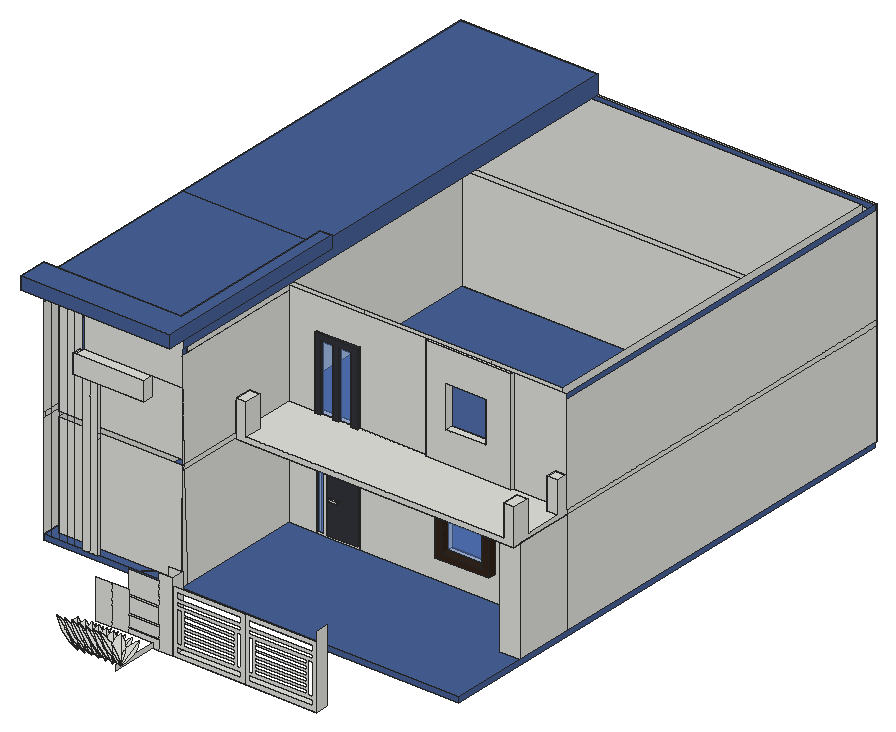
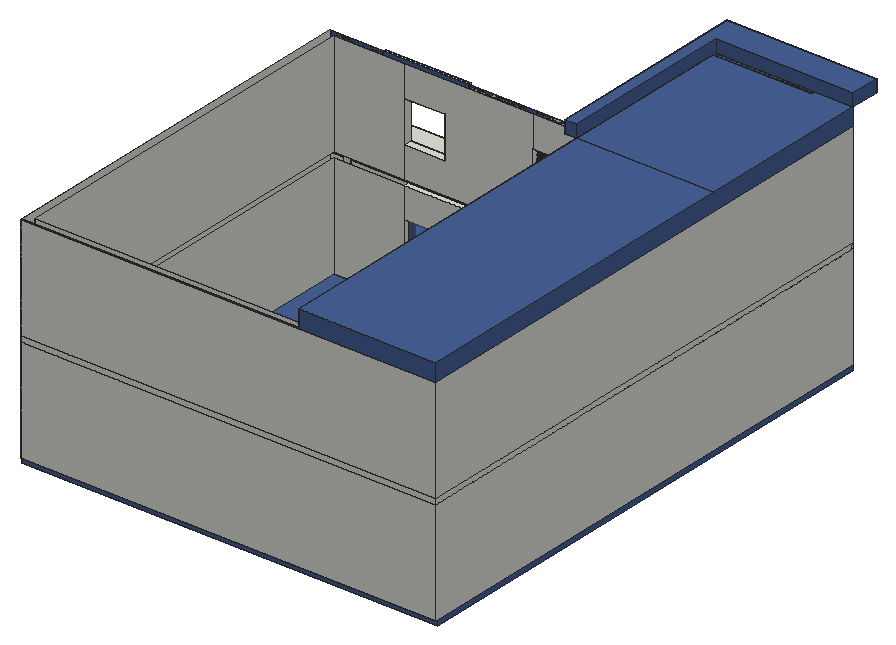
# SketchUp Ruby script. Lengths in inches.
U = 1.inch
M = Sketchup.active_model
def pt(a) = Geom::Point3d.new(a.map { |v| v * U })
def face(e, loops, mat)
  f = e.add_face(loops[0].map { |a| pt(a) })
  loops[1..].each { |l| e.add_face(l.map { |a| pt(a) }).erase! }
  f.material = f.back_material = mat if mat
  f
end
# faces: each face lists its corners as indices into pts; further lists are holes
def faces(e, pts, list, mat = nil) = list.each { |f| face(e, (f[0].is_a?(Array) ? f : [f]).map { |l| l.map { |i| pts[i] } }, mat) }
# xy, xz, yz: faces in a plane at the given z, y or x. An outline is a flat list of corners, or four numbers for a rectangle; further outlines are holes
def ring(l) = l.size == 4 ? [[l[0], l[1]], [l[2], l[1]], [l[2], l[3]], [l[0], l[3]]] : l.each_slice(2).to_a
def flat(e, list, mat, &to3) = list.each { |f| face(e, (f[0].is_a?(Array) ? f : [f]).map { |l| ring(l).map { |u, v| to3.(u, v) } }, mat) }
def xy(e, z, list, mat = nil) = flat(e, list, mat) { |x, y| [x, y, z] }
def xz(e, y, list, mat = nil) = flat(e, list, mat) { |x, z| [x, y, z] }
def yz(e, x, list, mat = nil) = flat(e, list, mat) { |y, z| [x, y, z] }
def lines(e, pts, list) = list.each { |a, b| e.add_line(pt(pts[a]), pt(pts[b])) }
# prism: a flat outline (further loops are holes) pulled along v
def prism(e, loops, v, mat = nil)
  f = face(e, loops, mat); d = Geom::Vector3d.new(v.map { |x| x * U })
  f.pushpull(f.normal.samedirection?(d) ? d.length : -d.length)
end
def box(e, o, s, mat = nil) = prism(e, [[o, [o[0] + s[0], o[1], o[2]], [o[0] + s[0], o[1] + s[1], o[2]], [o[0], o[1] + s[1], o[2]]]], [0, 0, s[2]], mat)
def at(x, y, z, deg = 0) = Geom::Transformation.translation(pt([x, y, z])) * Geom::Transformation.rotation(ORIGIN, Z_AXIS, deg.degrees)
def axes(o, x, y, z) = Geom::Transformation.new([*x, 0, *y, 0, *z, 0, *pt(o).to_a, 1])
def part(name) = M.definitions.add(name)
# library, detail: a bought-in or finely detailed component or shape, given as its bounding box
def library(name, o, s) = part(name).tap { |d| box(d.entities, o, s) }
def detail(e, o, s) = box(e.add_group.entities, o, s)
def put(e, d, t, mat = nil) = e.add_instance(d, t).tap { |i| i.material = mat if mat }
def group(e, t, mat = nil) = e.add_group.tap { |g| g.transformation = t; g.material = mat if mat }.entities
root = M.entities
M.materials.add("Teddy_HairLight").color = [51, 36, 26]
M.materials.add("[Formica Blue]").color = [71, 97, 152]
M.materials.add("[Formica Laminate Dark]").color = [50, 53, 60]
M.materials.add("[Translucent Glass Blue]").color = [100, 149, 237]
M.materials["[Translucent Glass Blue]"].alpha = 0.5
M.materials.add("[Translucent Glass Gold]").color = [255, 254, 26]
M.materials["[Translucent Glass Gold]"].alpha = 0.6
xy(root,-6,[[248.11,54.73,414.0625,69.27]])
xy(root,0,[[479.6,237.17,503.53,303.73]])
xy(root,29.625,[[359.09,294.73,420.53,303.73]],"Teddy_HairLight")
xy(root,36,[[366.125,294.73,389.29,303.73],[389.29,294.73,412.46,303.73]],"Teddy_HairLight")
xy(root,40.1875,[[232.4,300.42,240.9,303.73]])
xy(root,41.875,[[232.4,300.42,240.9,303.73]])
xy(root,47.5625,[[479.6,253.58,489.02,303.73]])
xy(root,84,[[366.125,294.73,389.29,303.73],[389.29,294.73,412.46,303.73]],"Teddy_HairLight")
xy(root,91.9375,[[359.09,294.73,420.53,303.73]],"Teddy_HairLight")
xy(root,114.125,[[479.6,253.58,489.02,303.73]])
xy(root,120,[[182.53,227.67,182.53,303.73,479.6,303.73,479.6,237.17,503.53,237.17,503.53,227.67],[489.02,237.17,503.53,303.73]])
xy(root,120.5,[[489.02,235.23,503.53,303.73]])
xy(root,126,[[194.53,227.67,491.53,227.67,491.53,247.23,503.53,247.23,503.53,290.6,491.53,290.6,491.53,302.6,503.53,302.6,503.53,303.73,264.52,303.73,264.52,300.85,257.03,300.85,257.03,303.73,243.03,303.73,243.03,300.85,236.35,300.85,236.35,303.73,221.92,303.73,221.92,300.85,214.94,300.85,214.94,303.73,182.53,303.73,182.53,247.23,194.53,247.23],[214.94,300.85,221.92,303.73],[236.35,300.85,243.03,303.73],[257.03,300.85,264.52,303.73]])
xy(root,161.75,[[182.53,227.67,194.53,247.23]])
xy(root,162,[[491.53,227.67,503.53,247.23],[491.53,290.6,503.53,302.6]])
xy(root,202.76,[[243.03,300.85,256.92,303.73]],"[Formica Laminate Dark]")
xy(root,203,[[221.92,300.85,236.28,303.73]],"[Formica Laminate Dark]")
xy(root,209.76,[[214.94,300.85,264.52,303.73]],"[Formica Laminate Dark]")
xz(root,54.73,[[224.41,-6,232.375,-6,232.375,5.02,196.97,5.02,196.97,-0.3125,224.41,-0.3125],[232.375,-6,248.11,74.8125],[[248.11,-6,331.08,66.46],[252.8,-1.3,252.8,61.76,326.38,61.76,326.38,54.54,252.8,54.54,252.8,51.52,326.38,51.52,326.38,47.54,252.8,47.54,252.8,44.52,258.3,44.52,258.3,8.6,260.27,8.6,260.27,13.25,319.99,13.25,319.99,8.6,252.8,8.6,252.8,5.58,326.38,5.58,326.38,8.6,321.96,8.6,321.96,44.52,326.38,44.52,326.38,-1.3],[260.27,14.87,319.99,19.57],[260.27,21.18,319.99,25.88],[260.27,27.49,319.99,32.19],[260.27,33.8,319.99,38.5],[260.27,40.12,319.99,44.52]],[[331.08,-6,414.0625,66.46],[342.96,27.49,342.96,32.19,402.49,32.19,402.49,33.8,342.96,33.8,342.96,38.5,402.49,38.5,402.49,27.49],[335.78,54.54,409.36,61.76],[335.78,-1.3,409.36,5.58],[335.78,47.54,409.36,51.52],[342.96,21.18,402.49,25.88],[342.96,14.87,402.49,19.57],[342.96,8.6,402.49,13.25],[342.96,40.12,402.49,44.52],[335.78,8.6,340.99,44.52],[404.46,8.6,409.36,44.52]],[159.72,-0.3125,178.2,45.33],
  [178.2,-0.3125,196.97,45.33],[196.97,5.02,232.375,6.44],[196.97,6.44,232.375,18.88],[196.97,18.88,232.375,20.57],[196.97,20.57,232.375,38.11],
  [196.97,38.11,232.375,40.33],[196.97,40.33,232.375,66]])
xz(root,69.27,[[232.375,-6,248.11,74.8125]])
xz(root,150.73,[[68.53,206.33,182.53,267.125]])
xz(root,227.67,[[182.53,120,503.53,120,503.53,162,491.53,162,491.53,126,194.53,126,194.53,161.75,182.53,161.75]])
xz(root,237.17,[[479.6,0,503.53,120]])
xz(root,247.23,[[182.53,126,194.53,161.75],[491.53,126,503.53,162]])
xz(root,253.58,[[479.6,47.5625,489.02,114.125]])
xz(root,290.6,[[491.53,126,503.53,162]])
xz(root,294.73,[[[359.09,29.625,420.53,91.9375],[366.125,36,412.46,84]]],"Teddy_HairLight")
xz(root,300.42,[[230.95,39.36,231.38,39.42,231.79,39.58,232.13,39.84,232.4,40.1875,240.9,40.1875,241.12,40.22,241.32,40.3,241.5,40.43,241.63,40.61,241.72,40.8125,241.75,41.03,241.72,41.25,241.63,41.45,241.5,41.63,241.32,41.76,241.12,41.85,240.9,41.875,232.4,41.875,232.15,42.2,231.81,42.47,231.41,42.64,230.98,42.7,230.54,42.64,230.14,42.48,229.79,42.22,229.53,41.875,229.36,41.47,229.3,41.04,229.35,40.61,229.51,40.21,229.78,39.86,230.12,39.59,230.52,39.42]])
xz(root,300.85,[[214.94,126,221.92,126,221.92,203,236.28,203,236.28,129.25,236.35,126,243.03,126,243.03,202.76,256.92,202.76,256.92,129.49,257.03,126,264.52,126,264.52,209.76,214.94,209.76]],"[Formica Laminate Dark]")
xz(root,302.6,[[491.53,126,503.53,162]])
xz(root,303.73,[[[214.94,0,225.66,84],[217.39,2.45,223.21,81.55]],[[225.66,0,264.52,84],[228.14,2.48,262.04,81.52]],[479.6,0,479.6,47.5625,489.02,47.5625,489.02,120,503.53,120,503.53,0],[[359.09,29.625,420.53,91.9375],[366.125,36,412.46,84]],[230.71,37.4,230.84,37.4,230.84,37.53,230.9,37.53,230.9,37.59,230.96,37.59,230.96,37.65,231.42,37.65,231.42,38.15,230.66,38.15,230.63,38.33,230.5625,38.5,230.45,38.64,230.31,38.75,230.14,38.82,229.96,38.85,229.78,38.82,229.61,38.75,229.47,38.64,229.36,38.5,229.29,38.33,229.27,38.15,229.29,37.97,229.36,37.8,229.47,37.66,229.61,37.55,229.78,37.48,229.96,37.46,230.14,37.48,230.31,37.55,230.44,37.65,230.71,37.65],
  [479.6,114.125,489.02,114.125,489.02,120.5,503.53,120.5,503.53,126,182.53,126,182.53,120,479.6,120],[489.02,120,503.53,120.5]])
xz(root,303.73,[[[228.14,2.48,262.04,81.52],[230.95,39.36,230.52,39.42,230.12,39.59,229.78,39.86,229.51,40.21,229.35,40.61,229.3,41.04,229.36,41.47,229.53,41.875,229.79,42.22,230.14,42.48,230.54,42.64,230.98,42.7,231.41,42.64,231.81,42.47,232.15,42.2,232.4,41.875,240.9,41.875,241.12,41.85,241.32,41.76,241.5,41.63,241.63,41.45,241.72,41.25,241.75,41.03,241.72,40.8125,241.63,40.61,241.5,40.43,241.32,40.3,241.12,40.22,240.9,40.1875,232.4,40.1875,232.13,39.84,231.79,39.58,231.38,39.42],[230.71,37.4,230.71,37.65,230.44,37.65,230.31,37.55,230.14,37.48,229.96,37.46,229.78,37.48,229.61,37.55,229.47,37.66,229.36,37.8,229.29,37.97,229.27,38.15,229.29,38.33,229.36,38.5,229.47,38.64,229.61,38.75,229.78,38.82,229.96,38.85,230.14,38.82,230.31,38.75,230.45,38.64,230.5625,38.5,230.63,38.33,230.66,38.15,231.42,38.15,231.42,37.65,230.96,37.65,230.96,37.59,230.9,37.59,230.9,37.53,230.84,37.53,230.84,37.4]]],"[Formica Laminate Dark]")
xz(root,303.73,[[217.39,2.45,223.21,81.55],[366.125,36,412.46,84],[221.92,126,236.35,126,236.28,129.25,236.28,203,221.92,203],[243.03,126,257.03,126,256.92,129.49,256.92,202.76,243.03,202.76]],"[Translucent Glass Blue]")
xz(root,750.73,[[23.53,120,503.53,126]])
yz(root,23.53,[[150.73,120,750.73,126]])
yz(root,182.53,[[150.73,120,153.18,120,152.93,126,150.73,126],[153.18,120,227.67,120,227.67,126,152.93,126],[150.73,126,152.93,126,150.73,177.86],[227.67,126,247.23,161.75],[150.73,177.86,150.73,206.33,150.5,183.15]])
yz(root,194.53,[[227.67,126,247.23,161.75]])
yz(root,214.94,[[300.85,126,303.73,209.76]],"[Formica Laminate Dark]")
yz(root,221.92,[[300.85,126,303.73,129.25],[300.85,129.25,303.73,203]],"[Formica Laminate Dark]")
yz(root,224.41,[[1.54,-6,54.73,-0.3125]])
yz(root,236.28,[[300.85,129.25,303.73,203]],"[Formica Laminate Dark]")
yz(root,243.03,[[300.85,126,303.73,129.49],[300.85,129.49,303.73,202.76]],"[Formica Laminate Dark]")
yz(root,248.11,[[54.73,-6,69.27,74.8125]])
yz(root,256.92,[[300.85,129.49,303.73,202.76]],"[Formica Laminate Dark]")
yz(root,264.52,[[300.85,126,303.73,209.76]],"[Formica Laminate Dark]")
yz(root,359.09,[[294.73,29.625,303.73,91.9375]],"Teddy_HairLight")
yz(root,366.125,[[294.73,36,303.73,60],[294.73,60,303.73,84]],"Teddy_HairLight")
yz(root,412.46,[[294.73,36,303.73,60],[294.73,60,303.73,84]],"Teddy_HairLight")
yz(root,414.0625,[[54.73,-6,69.27,77.75]])
yz(root,420.53,[[294.73,29.625,303.73,91.9375]],"Teddy_HairLight")
yz(root,479.6,[[237.17,0,237.17,120,303.73,120,303.73,114.125,253.58,114.125,253.58,47.5625,303.73,47.5625,303.73,0]],"[Translucent Glass Gold]")
yz(root,489.02,[[253.58,47.5625,303.73,114.125]])
yz(root,491.53,[[227.67,126,247.23,162],[290.6,126,302.6,162]])
yz(root,503.53,[[237.17,0,303.73,120],[227.67,120,235.23,120,235.23,120.5,303.73,120.5,303.73,126,302.6,126,302.6,162,290.6,162,290.6,126,247.23,126,247.23,162,227.67,162],[235.23,120,303.73,120.5],[303.73,120,750.73,126]])
p = [[204.65,4.95,22.91],[203.55,5.4375,25.45],[217.13,5.38,9.44],[217.26,5.28,9.03],[218.46,4.85,6.54],[220.07,4.64,4.13],
  [222.0625,4.66,1.84],[224.41,4.89,-0.3125],[227.08,5.34,-2.29],[224.34,4.86,-0.3],[221.72,4.47,1.77],[219.24,4.17,3.9],
  [216.89,3.96,6.1],[214.6875,3.83,8.36],[212.625,3.8,10.68],[210.72,3.85,13.04],[208.96,3.99,15.45],[207.36,4.22,17.91],
  [205.93,4.54,20.39],[216.12,6.76,14.12],[216.15,7.26,15.36],[216.51,7.29,15.01],[218.6,7.33,12.68],[220.5,7.27,10.3],
  [222.22,7.1,7.86],[223.74,6.82,5.37],[225.06,6.43,2.85],[226.17,5.9375,0.29],[216.47,5.91,11.57],[220.75,13.54,25.94],
  [225.96,6.8,2.72],[225.99,6.6,2.19],[226.39,5.9,-0.06],[216.19,7.79,16.65],[216.71,9,19.13],[217.65,10.38,21.53],
  [219,11.9,23.81],[225.87,7.43,4.43],[226.04,8.38,6.66],[226.49,9.45,8.84],[227.23,10.63,10.98],[228.03,11.64,12.59],
  [228.2,11.47,11.97],[228.625,10.71,9.55],[228.8,9.84,7.13],[228.74,8.86,4.73],[228.43,7.78,2.35],[227.875,6.61,0],
  [234.93,17.84,20.29],[237.18,19.47,21.79],[228.25,11.91,13.04],[229.54,13.28,15.01],[231.09,14.74,16.89],[232.89,16.26,18.66],
  [237.49,18.74,19.58],[237.59,17.92,17.38],[237.46,17,15.2],[237.13,15.99,13.04],[236.58,14.9,10.91],[235.82,13.73,8.82],
  [234.85,12.49,6.79],[233.68,11.17,4.82],[232.3125,9.8,2.92],[230.75,8.36,1.09],[229.01,6.87,-0.65],[196.51,4.79,22.99],
  [195.41,5.29,25.53],[208.99,5.23,9.52],[209.11,5.125,9.11],[210.32,4.7,6.62],[211.93,4.49,4.21],[213.92,4.5,1.92],
  [216.27,4.74,-0.23],[218.94,5.19,-2.21],[216.2,4.71,-0.22],[213.58,4.32,1.85],[211.1,4.02,3.98],[208.75,3.8,6.18],
  [206.54,3.68,8.44],[204.48,3.64,10.76],[202.57,3.7,13.12],[200.82,3.84,15.53],[199.22,4.07,17.99],[197.78,4.39,20.47],
  [212.61,13.39,26.02],[217.82,6.64,2.8],[217.84,6.45,2.27],[218.25,5.75,0.02],[218.03,5.78,0.37],[216.92,6.28,2.92],
  [215.6,6.67,5.45],[214.08,6.95,7.9375],[212.36,7.12,10.375],[210.46,7.18,12.76],[208.37,7.13,15.09],[208.01,7.11,15.44],
  [208.05,7.64,16.73],[208.57,8.85,19.21],[209.51,10.23,21.61],[210.86,11.75,23.89],[207.97,6.6,14.2],[208.33,5.76,11.65],
  [217.72,7.28,4.51],[217.89,8.23,6.74],[218.35,9.3,8.92],[219.09,10.48,11.05],[219.89,11.48,12.67],[220.0625,11.32,12.05],
  [220.48,10.56,9.63],[220.66,9.6875,7.21],[220.59,8.71,4.81],[220.28,7.63,2.43],[219.73,6.45,0.08],[226.78,17.6875,20.37],
  [229.04,19.3125,21.87],[220.11,11.76,13.12],[221.4,13.13,15.09],[222.95,14.58,16.97],[224.75,16.11,18.73],[229.35,18.59,19.66],
  [229.44,17.76,17.46],[229.32,16.85,15.28],[228.99,15.84,13.11],[228.4375,14.75,10.99],[227.68,13.58,8.9],[226.71,12.34,6.87],
  [225.54,11.02,4.9],[224.17,9.64,3],[222.61,8.21,1.17],[220.86,6.72,-0.57],[180.23,4.49,23.15],[179.12,4.98,25.69],
  [192.7,4.92,9.68],[192.83,4.82,9.27],[194.03,4.4,6.78],[195.64,4.1875,4.37],[197.63,4.2,2.08],[199.98,4.43,-0.07],
  [202.66,4.88,-2.06],[199.91,4.41,-0.0625],[197.3,4.02,2],[194.81,3.71,4.14],[192.47,3.5,6.34],[190.26,3.375,8.6],
  [188.2,3.34,10.92],[186.29,3.39,13.28],[184.53,3.54,15.69],[182.9375,3.77,18.14],[181.5,4.08,20.63],[188.37,4.64,23.07],
  [187.26,5.13,25.61],[200.84,5.08,9.6],[200.97,4.97,9.19],[202.18,4.55,6.7],[203.79,4.34,4.29],[205.78,4.35,2],
  [208.125,4.58,-0.15],[210.8,5.03,-2.14],[208.06,4.56,-0.14],[205.44,4.17,1.92],[202.96,3.87,4.06],[200.61,3.65,6.26],
  [198.4,3.53,8.52],[196.34,3.49,10.84],[194.43,3.55,13.2],[192.68,3.6875,15.61],[191.08,3.92,18.07],[189.64,4.24,20.55],
  [196.33,13.09,26.18],[201.53,6.34,2.96],[201.56,6.14,2.43],[201.97,5.44,0.18],[201.75,5.48,0.53],[200.63,5.97,3.08],
  [199.3125,6.36,5.61],[197.79,6.64,8.1],[196.08,6.8125,10.54],[194.17,6.88,12.92],[192.08,6.83,15.24],[191.73,6.81,15.6],
  [191.77,7.33,16.89],[192.28,8.55,19.37],[193.22,9.92,21.77],[194.58,11.44,24.05],[191.6875,6.3,14.36],[192.04,5.46,11.81],
  [201.44,6.97,4.67],[201.61,7.93,6.9],[202.07,9,9.08],[202.81,10.18,11.21],[203.61,11.18,12.83],[203.78,11.01,12.21],
  [204.2,10.25,9.79],[204.375,9.38,7.37],[204.31,8.41,4.96],[204,7.33,2.58],[203.45,6.15,0.24],[210.5,17.38,20.53],
  [212.76,19.01,22.03],[203.83,11.46,13.28],[205.12,12.83,15.25],[206.67,14.28,17.13],[208.47,15.8,18.89],[213.07,18.28,19.82],
  [213.16,17.46,17.62],[213.04,16.54,15.43],[212.7,15.54,13.27],[212.15,14.45,11.15],[211.39,13.28,9.0625],[210.43,12.03,7.03],
  [209.26,10.72,5.06],[207.89,9.34,3.16],[206.33,7.9,1.33],[204.58,6.42,-0.41],[199.83,6.45,14.28],[199.87,6.96,15.52],
  [200.23,6.98,15.17],[202.32,7.03,12.84],[204.22,6.97,10.46],[205.94,6.79,8.02],[207.45,6.51,5.53],[208.77,6.125,3],
  [209.89,5.63,0.45],[200.1875,5.61,11.73],[204.47,13.24,26.1],[209.67,6.49,2.88],[209.7,6.29,2.35],[210.11,5.6,0.1],
  [199.91,7.49,16.8125],[200.42,8.7,19.29],[201.36,10.07,21.6875],[202.72,11.59,23.97],[209.58,7.125,4.59],[209.75,8.08,6.82],
  [210.21,9.15,9],[210.95,10.33,11.13],[211.75,11.33,12.75],[211.92,11.17,12.13],[212.34,10.41,9.71],[212.52,9.54,7.29],
  [212.45,8.56,4.88],[212.14,7.48,2.51],[211.59,6.3,0.16],[218.64,17.53,20.45],[220.9,19.16,21.95],[211.97,11.61,13.2],
  [213.26,12.98,15.17],[214.81,14.43,17.05],[216.61,15.95,18.8125],[221.21,18.43,19.74],[221.3,17.61,17.54],[221.18,16.7,15.35],
  [220.84,15.69,13.19],[220.3,14.6,11.07],[219.54,13.43,8.98],[218.57,12.18,6.95],[217.4,10.87,4.98],[216.03,9.49,3.08],
  [214.47,8.06,1.25],[212.72,6.57,-0.49],[172.09,4.34,23.23],[170.98,4.83,25.77],[184.56,4.77,9.76],[184.6875,4.67,9.35],
  [185.89,4.24,6.86],[187.5,4.04,4.45],[189.49,4.05,2.16],[191.84,4.28,0],[194.51,4.73,-1.98],[191.77,4.25,0.02],
  [189.16,3.86,2.08],[186.67,3.5625,4.22],[184.33,3.35,6.42],[182.12,3.22,8.68],[180.06,3.1875,10.99],[178.15,3.24,13.36],
  [176.39,3.38,15.77],[174.8,3.61,18.22],[173.36,3.93,20.71],[183.55,6.15,14.4375],[183.59,6.66,15.68],[183.94,6.68,15.32],
  [186.03,6.73,13],[187.9375,6.66,10.61],[189.65,6.49,8.17],[191.17,6.21,5.6875],[192.49,5.82,3.16],[193.61,5.33,0.6],
  [183.9,5.31,11.89],[188.1875,12.9375,26.26],[193.39,6.1875,3.04],[193.42,5.99,2.51],[193.82,5.29,0.26],[183.625,7.18,16.97],
  [184.14,8.39,19.45],[185.08,9.77,21.85],[186.43,11.29,24.125],[193.3,6.82,4.75],[193.47,7.77,6.98],[193.93,8.84,9.16],
  [194.67,10.02,11.29],[195.46,11.03,12.91],[195.64,10.86,12.29],[196.06,10.1,9.87],[196.23,9.23,7.45],[196.17,8.25,5.04],
  [195.86,7.18,2.66],[195.31,6,0.32],[202.36,17.23,20.61],[204.62,18.86,22.11],[195.68,11.3,13.35],[196.97,12.68,15.33],
  [198.52,14.13,17.21],[200.32,15.65,18.97],[204.92,18.13,19.9],[205.02,17.31,17.7],[204.9,16.39,15.51],[204.56,15.39,13.35],
  [204.01,14.3,11.22],[203.25,13.125,9.14],[202.28,11.88,7.11],[201.11,10.57,5.14],[199.75,9.1875,3.23],[198.19,7.75,1.41],
  [196.4375,6.26,-0.33],[163.94,4.1875,23.31],[162.84,4.68,25.85],[176.42,4.62,9.84],[176.55,4.52,9.43],[177.75,4.09,6.9375],
  [179.36,3.88,4.53],[181.35,3.9,2.24],[183.7,4.13,0.08],[186.37,4.58,-1.9],[183.63,4.1,0.1],[181.02,3.71,2.16],
  [178.53,3.41,4.3],[176.18,3.2,6.5],[173.98,3.07,8.76],[171.92,3.04,11.07],[170.01,3.09,13.44],[168.25,3.23,15.85],
  [166.65,3.46,18.3],[165.22,3.78,20.79],[180.04,12.78,26.34],[185.25,6.04,3.12],[185.28,5.84,2.59],[185.68,5.14,0.34],
  [185.46,5.18,0.68],[184.35,5.67,3.24],[183.03,6.06,5.77],[181.51,6.34,8.25],[179.79,6.51,10.69],[177.89,6.57,13.08],
  [175.8,6.53,15.4],[175.44,6.5,15.76],[175.48,7.03,17.05],[176,8.24,19.53],[176.9375,9.62,21.93],[178.29,11.14,24.2],
  [175.41,6,14.52],[175.76,5.16,11.96],[185.16,6.67,4.83],[185.33,7.62,7.05],[185.78,8.69,9.24],[186.52,9.87,11.37],
  [187.32,10.875,12.99],[187.49,10.71,12.37],[187.91,9.95,9.95],[188.09,9.08,7.53],[188.03,8.1,5.12],[187.72,7.02,2.74],
  [187.16,5.85,0.4],[194.22,17.08,20.6875],[196.47,18.71,22.19],[187.54,11.15,13.43],[188.83,12.52,15.41],[190.38,13.98,17.29],
  [192.18,15.5,19.05],[196.78,17.98,19.98],[196.875,17.16,17.78],[196.75,16.24,15.59],[196.42,15.23,13.43],[195.87,14.14,11.3],
  [195.11,12.97,9.22],[194.14,11.73,7.1875],[192.97,10.41,5.22],[191.6,9.04,3.3125],[190.04,7.6,1.49],[188.3,6.11,-0.25],
  [155.8,4.03,23.39],[154.7,4.53,25.93],[168.28,4.47,9.92],[168.4,4.37,9.51],[169.61,3.94,7.02],[171.22,3.73,4.61],
  [173.21,3.74,2.32],[175.56,3.98,0.16],[178.23,4.43,-1.82],[175.49,3.95,0.18],[172.875,3.5625,2.24],[170.39,3.26,4.38],
  [168.04,3.05,6.58],[165.84,2.92,8.84],[163.77,2.88,11.15],[161.86,2.9375,13.52],[160.11,3.08,15.93],[158.51,3.31,18.38],
  [157.07,3.63,20.87],[171.9,12.63,26.42],[177.11,5.88,3.2],[177.13,5.6875,2.67],[177.54,4.99,0.42],[177.32,5.02,0.76],
  [176.21,5.52,3.32],[174.89,5.91,5.85],[173.37,6.1875,8.33],[171.65,6.36,10.77],[169.75,6.42,13.16],[167.66,6.375,15.48],
  [167.3,6.35,15.84],[167.34,6.88,17.13],[167.86,8.09,19.61],[168.8,9.47,22],[170.15,10.99,24.28],[167.26,5.84,14.6],
  [167.62,5,12.04],[177.02,6.52,4.91],[177.18,7.47,7.13],[177.64,8.54,9.32],[178.38,9.72,11.45],[179.18,10.72,13.07],
  [179.35,10.56,12.45],[179.77,9.8,10.03],[179.95,8.93,7.61],[179.88,7.95,5.2],[179.57,6.87,2.82],[179.02,5.69,0.48],
  [186.08,16.93,20.77],[188.33,18.55,22.26],[179.4,11,13.51],[180.69,12.37,15.49],[182.24,13.82,17.37],[184.04,15.35,19.13],
  [188.64,17.83,20.06],[188.73,17,17.86],[188.61,16.09,15.67],[188.28,15.08,13.51],[187.73,13.99,11.38],[186.97,12.82,9.3],
  [186,11.58,7.27],[184.83,10.26,5.3],[183.46,8.88,3.39],[181.9,7.45,1.57],[180.15,5.96,-0.17],[227.54,12.12,14.38],
  [222.56,13.5,23.73],[224.14,13.34,21.46],[225.51,13.05,19.14],[226.64,12.64,16.78],[219.4,11.96,14.46],[214.41,13.35,23.8125],
  [216,13.1875,21.54],[217.36,12.9,19.22],[218.5,12.49,16.86],[211.26,11.8125,14.54],[206.27,13.2,23.89],[207.86,13.04,21.62],
  [209.22,12.75,19.3],[210.36,12.34,16.9375],[194.97,11.51,14.7],[189.99,12.9,24.05],[191.57,12.73,21.78],[192.9375,12.44,19.46],
  [194.07,12.04,17.1],[203.12,11.66,14.62],[198.13,13.05,23.97],[199.72,12.88,21.7],[201.08,12.6,19.38],[202.21,12.1875,17.02],
  [186.83,11.36,14.78],[181.85,12.74,24.13],[183.43,12.58,21.86],[184.8,12.29,19.54],[185.93,11.88,17.17],[178.6875,11.2,14.86],
  [173.7,12.59,24.21],[175.29,12.43,21.9375],[176.65,12.14,19.62],[177.79,11.73,17.25],[206.45,6.02,23.54],[209.21,6.5,21.54],
  [211.81,6.87,19.44],[214.24,7.13,17.26],[198.31,5.87,23.62],[201.0625,6.35,21.62],[203.66,6.72,19.52],[206.1,6.98,17.34],
  [190.17,5.72,23.7],[192.92,6.19,21.69],[195.52,6.57,19.6],[197.96,6.83,17.42],[182.02,5.57,23.78],[184.78,6.04,21.77],
  [187.38,6.41,19.68],[189.82,6.68,17.5],[165.74,5.26,23.9375],[168.5,5.74,21.93],[171.1,6.11,19.84],[173.53,6.37,17.66],
  [173.88,5.41,23.86],[176.64,5.89,21.85],[179.24,6.26,19.76],[181.68,6.52,17.58],[157.6,5.11,24.02],[160.35,5.59,22.01],
  [162.95,5.96,19.92],[165.39,6.22,17.74],[230.12,303.73,39.59],[230.52,303.73,39.42],[230.52,300.42,39.42],[230.12,300.42,39.59],
  [230.95,303.73,39.36],[230.95,300.42,39.36],[231.38,303.73,39.42],[231.38,300.42,39.42],[231.79,303.73,39.58],[231.79,300.42,39.58],
  [229.78,303.73,39.86],[229.78,300.42,39.86],[232.13,303.73,39.84],[232.13,300.42,39.84],[232.4,303.73,40.1875],[232.4,300.42,40.1875],
  [229.51,303.73,40.21],[229.51,300.42,40.21],[229.35,303.73,40.61],[229.35,300.42,40.61],[240.9,303.73,40.1875],[241.12,303.73,40.22],
  [241.12,300.42,40.22],[240.9,300.42,40.1875],[241.32,303.73,40.3],[241.32,300.42,40.3],[241.5,303.73,40.43],[241.5,300.42,40.43],
  [241.63,303.73,40.61],[241.63,300.42,40.61],[229.3,303.73,41.04],[229.3,300.42,41.04],[241.72,303.73,40.8125],[241.72,300.42,40.8125],
  [241.75,303.73,41.03],[241.75,300.42,41.03],[229.36,303.73,41.47],[229.36,300.42,41.47],[241.72,303.73,41.25],[241.72,300.42,41.25],
  [241.63,303.73,41.45],[241.63,300.42,41.45],[229.53,303.73,41.875],[229.53,300.42,41.875],[241.5,303.73,41.63],[241.5,300.42,41.63],
  [241.32,303.73,41.76],[241.32,300.42,41.76],[241.12,303.73,41.85],[240.9,303.73,41.875],[240.9,300.42,41.875],[241.12,300.42,41.85],
  [229.79,303.73,42.22],[229.79,300.42,42.22],[232.4,303.73,41.875],[232.15,303.73,42.2],[232.15,300.42,42.2],[232.4,300.42,41.875],
  [230.14,303.73,42.48],[230.14,300.42,42.48],[231.81,303.73,42.47],[231.81,300.42,42.47],[230.54,303.73,42.64],[230.54,300.42,42.64],
  [231.41,303.73,42.64],[231.41,300.42,42.64],[230.98,303.73,42.7],[230.98,300.42,42.7],[236.28,303.73,129.25],[236.35,303.73,126],
  [236.35,300.85,126],[236.28,300.85,129.25],[256.92,303.73,129.49],[257.03,303.73,126],[257.03,300.85,126],[256.92,300.85,129.49],
  [182.53,148.73,0],[182.53,150.5,183.15],[182.53,150.73,0],[182.53,150.73,120],[182.53,153.18,120],[182.53,158.26,0.32]]
faces(root,p,[[0,1,2,3,4,5,6,7,8,9,10,11,12,13,14,15,16,17,18],[3,2,8,7,6,5,4],[19,20,21,22,23,24,25,26,27,8,2,28],[29,30,31,32,8,27,26,25,24,23,22,21,20,33,34,35,36],[8,30,37,38,39,40,41,42,43,44,45,46,47],[30,8,32,31],[48,49,8,47,46,45,44,43,42,41,50,51,52,53],[8,49,54,55,56,57,58,59,60,61,62,63,64],
  [65,66,67,68,69,70,71,72,73,74,75,76,77,78,79,80,81,82,83],[68,67,73,72,71,70,69],[84,85,86,87,73,88,89,90,91,92,93,94,95,96,97,98,99],[100,95,94,93,92,91,90,89,88,73,67,101],[73,85,102,103,104,105,106,107,108,109,110,111,112],[85,73,87,86],[113,114,73,112,111,110,109,108,107,106,115,116,117,118],[73,114,119,120,121,122,123,124,125,126,127,128,129],
  [130,131,132,133,134,135,136,137,138,139,140,141,142,143,144,145,146,147,148],[149,150,151,152,153,154,155,156,157,158,159,160,161,162,163,164,165,166,167],[133,132,138,137,136,135,134],[152,151,157,156,155,154,153],[168,169,170,171,138,172,173,174,175,176,177,178,179,180,181,182,183],[184,179,178,177,176,175,174,173,172,138,132,185],[138,169,186,187,188,189,190,191,192,193,194,195,196],[169,138,171,170],
  [197,198,138,196,195,194,193,192,191,190,199,200,201,202],[138,198,203,204,205,206,207,208,209,210,211,212,213],[214,215,216,217,218,219,220,221,222,157,151,223],[224,225,226,227,157,222,221,220,219,218,217,216,215,228,229,230,231],[157,225,232,233,234,235,236,237,238,239,240,241,242],[225,157,227,226],[243,244,157,242,241,240,239,238,237,236,245,246,247,248],[157,244,249,250,251,252,253,254,255,256,257,258,259],
  [260,261,262,263,264,265,266,267,268,269,270,271,272,273,274,275,276,277,278],[263,262,268,267,266,265,264],[279,280,281,282,283,284,285,286,287,268,262,288],[289,290,291,292,268,287,286,285,284,283,282,281,280,293,294,295,296],[268,290,297,298,299,300,301,302,303,304,305,306,307],[290,268,292,291],[308,309,268,307,306,305,304,303,302,301,310,311,312,313],[268,309,314,315,316,317,318,319,320,321,322,323,324],
  [325,326,327,328,329,330,331,332,333,334,335,336,337,338,339,340,341,342,343],[328,327,333,332,331,330,329],[344,345,346,347,333,348,349,350,351,352,353,354,355,356,357,358,359],[360,355,354,353,352,351,350,349,348,333,327,361],[345,333,347,346],[333,345,362,363,364,365,366,367,368,369,370,371,372],[373,374,333,372,371,370,369,368,367,366,375,376,377,378],[333,374,379,380,381,382,383,384,385,386,387,388,389],
  [390,391,392,393,394,395,396,397,398,399,400,401,402,403,404,405,406,407,408],[393,392,398,397,396,395,394],[409,410,411,412,398,413,414,415,416,417,418,419,420,421,422,423,424],[425,420,419,418,417,416,415,414,413,398,392,426],[398,410,427,428,429,430,431,432,433,434,435,436,437],[410,398,412,411],[438,439,398,437,436,435,434,433,432,431,440,441,442,443],[398,439,444,445,446,447,448,449,450,451,452,453,454],
  [455,41,40,39,38,37,30,29,456,457,458,459],[460,106,105,104,103,102,85,84,461,462,463,464],[465,236,235,234,233,232,225,224,466,467,468,469],[470,301,300,299,298,297,290,289,471,472,473,474],[475,190,189,188,187,186,169,168,476,477,478,479],[480,366,365,364,363,362,345,344,481,482,483,484],[485,431,430,429,428,427,410,409,486,487,488,489],[2,1,490,491,492,493,20,19,28],
  [67,66,494,495,496,497,95,100,101],[151,150,498,499,500,501,215,214,223],[132,131,502,503,504,505,179,184,185],[327,326,506,507,508,509,355,360,361],[262,261,510,511,512,513,280,279,288],[392,391,514,515,516,517,420,425,426],[518,519,520,521],[519,522,523,520],
  [522,524,525,523],[524,526,527,525],[528,518,521,529],[526,530,531,527],[530,532,533,531],[534,528,529,535],[536,534,535,537],[538,539,540,541],
  [539,542,543,540],[542,544,545,543],[544,546,547,545],[548,536,537,549],[546,550,551,547],[550,552,553,551],[554,548,549,555],[552,556,557,553],
  [556,558,559,557],[560,554,555,561],[558,562,563,559],[562,564,565,563],[566,567,568,569],[564,566,569,565],[570,560,561,571],[572,573,574,575],
  [576,570,571,577],[573,578,579,574],[580,576,577,581],[578,582,583,579],[584,580,581,585],[582,584,585,583]])
faces(root,p,[[586,587,588,589],[590,591,592,593]],"[Formica Laminate Dark]")
lines(root,p,[[594,595],[596,597],[598,599]])
g1 = group(root,at(581.5625,-817.79,0),"[Formica Blue]")
xy(g1,240,[[-513.03,974.52,-399.03,975.21]])
xy(g1,246,[[-513.03,970.52,-399.03,974.52],[-513.03,974.52,-399.03,975.21]])
xy(g1,267.125,[[-558.03,933.08,-558.03,966.52,-399.03,966.52,-399.03,1166.93,-385.65,1166.93,-385.65,933.08],[-558.03,966.52,-513.03,966.52,-513.03,970.52,-399.03,970.52,-399.03,1166.93,-558.03,1166.93],[-513.03,966.52,-399.03,970.52],[-558.03,1166.93,-399.03,1568.52]])
xy(g1,281.625,[[-558.03,933.08,-385.65,933.08,-385.65,1166.93,-399.03,1166.93,-399.03,966.52,-558.03,966.52]])
xz(g1,933.08,[[-558.03,267.125,-385.65,281.625]])
xz(g1,966.52,[[-558.03,267.125,-399.03,281.625]])
xz(g1,970.52,[[-513.03,246,-399.03,267.125]])
xz(g1,974.52,[[-513.03,240,-399.03,246]])
xz(g1,975.21,[[-513.03,240,-399.03,246]])
xz(g1,1166.93,[[-399.03,267.125,-385.65,281.625]])
xz(g1,1568.52,[[-558.03,246,-399.03,267.125]])
yz(g1,-558.03,[[966.52,246,1568.52,267.125],[933.08,267.125,966.52,281.625]])
yz(g1,-513.03,[[968.52,240,974.52,246],[974.52,240,975.21,246],[966.52,246,970.52,267.125]])
yz(g1,-399.03,[[968.52,240,974.52,246],[974.52,240,975.21,246],[970.52,246,1568.52,267.125],[966.52,267.125,1166.93,281.625]])
yz(g1,-385.65,[[933.08,267.125,1166.93,281.625]])
p = [[-549.03,966.52,240],[-549.03,966.52,267.125],[-522.03,966.52,246],[-522.03,966.52,267.125]]
lines(g1,p,[[0,1],[2,3]])
g2 = group(g1,at(0,0,0))
box(g2,[-558.03,966.52,-6],[480,600,6])
xz(g2,1121.52,[[-399.03,240,-78.03,246]])
xz(g2,1566.52,[[-558.03,240,-78.03,246]])
yz(g2,-558.03,[[966.52,240,1566.52,246]])
yz(g2,-78.03,[[1121.52,240,1566.52,246]])
p = [[-399.03,966.52,240],[-399.03,1121.52,240]]
lines(g2,p,[[0,1]])
g3 = group(root,at(23.53,147.48,0))
xy(g3,0,[[0,1.25,63,1.25,63,3.25,159,3.25,159,156.25,191.41,156.25,191.41,162.25,153,162.25,153,12.25,9,12.25,9,594.25,471,594.25,471,162.25,240.99,162.25,240.99,156.25,480,156.25,480,603.25,0,603.25],[191.41,156.25,240.99,162.25]])
xy(g3,36,[[342.59,156.25,388.93,162.25]])
xy(g3,84,[[191.41,156.25,240.99,162.25],[342.59,156.25,388.93,162.25]])
xy(g3,120,[[240.99,156.25,388.93,162.25]])
xy(g3,126,[[319.5,153,418.58,156.25],[191.41,156.25,240.99,162.25]])
xy(g3,162,[[342.59,153,388.93,162.25]])
xy(g3,184.95,[[42.04,-8.75,45,1.25],[45,-8.75,45,1.25,63,1.25,63,3.25,123.73,3.25,123.73,-8.75]])
xy(g3,206.33,[[45,-8.75,123.73,3.25]])
xy(g3,206.39,[[42.04,-8.75,45,1.25]])
xy(g3,209.76,[[191.41,156.25,240.99,162.25]])
xy(g3,210,[[342.59,153,388.93,162.25]])
xy(g3,246,[[319.5,153,418.58,156.25]])
xz(g3,-8.75,[[42.04,184.95,123.73,184.95,123.73,206.33,45,206.33,45,206.39,42.04,206.39]])
xz(g3,1.25,[[45,0,54,184.95],[54,0,63,184.95]])
xz(g3,12.25,[[9,0,153,120],[9,126,153,246]])
xz(g3,153,[[[319.5,126,418.58,246],[342.59,162,388.93,210]]])
xz(g3,156.25,[[[159,0,191.41,0,191.41,84,240.99,84,240.99,0,480,0,480,120,159,120],[342.59,36,388.93,84]],[159,126,191.41,126,191.41,209.76,240.99,209.76,240.99,126,319.5,126,319.5,246,159,246],[418.58,126,480,246]])
xz(g3,162.25,[[153,0,153,120,240.99,120,240.99,84,191.41,84,191.41,0],[240.99,0,240.99,120,388.93,120,388.93,84,342.59,84,342.59,36,388.93,36,388.93,0],[388.93,0,471,120],[153,126,153,246,240.99,246,240.99,209.76,191.41,209.76,191.41,126],[240.99,126,240.99,246,388.93,246,388.93,210,342.59,210,342.59,162,388.93,162,388.93,126],
  [388.93,126,471,246]])
xz(g3,594.25,[[9,0,471,120],[9,126,471,246]])
xz(g3,603.25,[[0,0,480,120],[0,126,480,246]])
yz(g3,0,[[1.25,0,603.25,120],[1.25,120,3.25,126],[1.25,126,603.25,246]])
yz(g3,9,[[12.25,0,594.25,120],[12.25,126,594.25,246]])
yz(g3,42.04,[[-8.75,184.95,1.25,206.39]])
yz(g3,45,[[-8.75,206.33,1.25,206.39],[1.25,206.33,3.25,246]],"[Formica Blue]")
yz(g3,63,[[1.25,0,3.25,120],[1.25,120,3.25,126],[1.25,126,3.25,184.95]])
yz(g3,123.73,[[-8.75,184.95,3.25,206.33]])
yz(g3,153,[[12.25,0,162.25,120],[12.25,126,162.25,246]])
yz(g3,159,[[3.25,0,156.25,120],[3.25,126,156.25,246]])
yz(g3,191.41,[[156.25,0,162.25,84],[156.25,126,162.25,209.76]])
yz(g3,240.99,[[156.25,0,162.25,84],[156.25,126,162.25,209.76]])
yz(g3,319.5,[[153,126,156.25,246]])
yz(g3,342.59,[[156.25,36,162.25,84],[153,162,162.25,210]])
yz(g3,388.93,[[156.25,36,162.25,84],[153,162,162.25,210]])
yz(g3,418.58,[[153,126,156.25,246]])
yz(g3,471,[[162.25,0,594.25,120],[162.25,126,594.25,246]])
yz(g3,480,[[156.25,0,603.25,120],[156.25,126,603.25,246]])
p = [[159,3.25,0],[159,0,0],[159,3.25,126],[159,3.25,120],[27,1.25,0],[27,1.25,246],
  [9,1.25,0],[9,1.25,246],[18,1.25,246],[18,1.25,0],[36,1.25,246],[36,1.25,0]]
lines(g3,p,[[0,1],[2,3],[4,5],[6,7],[8,9],[10,11]])
